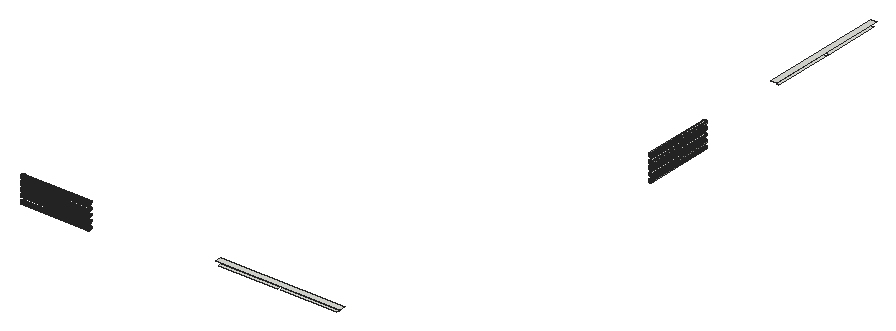
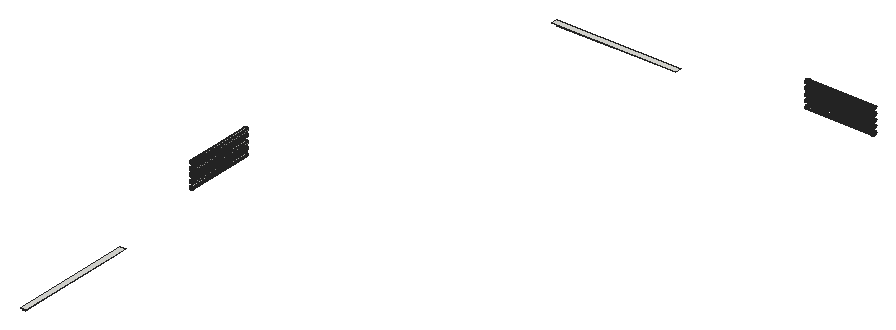
# SketchUp Ruby script. Lengths in inches.
U = 1.inch
M = Sketchup.active_model
def pt(a) = Geom::Point3d.new(a.map { |v| v * U })
def face(e, loops, mat)
  f = e.add_face(loops[0].map { |a| pt(a) })
  loops[1..].each { |l| e.add_face(l.map { |a| pt(a) }).erase! }
  f.material = f.back_material = mat if mat
  f
end
# faces: each face lists its corners as indices into pts; further lists are holes
def faces(e, pts, list, mat = nil) = list.each { |f| face(e, (f[0].is_a?(Array) ? f : [f]).map { |l| l.map { |i| pts[i] } }, mat) }
# xy, xz, yz: faces in a plane at the given z, y or x. An outline is a flat list of corners, or four numbers for a rectangle; further outlines are holes
def ring(l) = l.size == 4 ? [[l[0], l[1]], [l[2], l[1]], [l[2], l[3]], [l[0], l[3]]] : l.each_slice(2).to_a
def flat(e, list, mat, &to3) = list.each { |f| face(e, (f[0].is_a?(Array) ? f : [f]).map { |l| ring(l).map { |u, v| to3.(u, v) } }, mat) }
def xy(e, z, list, mat = nil) = flat(e, list, mat) { |x, y| [x, y, z] }
def xz(e, y, list, mat = nil) = flat(e, list, mat) { |x, z| [x, y, z] }
def yz(e, x, list, mat = nil) = flat(e, list, mat) { |y, z| [x, y, z] }
def lines(e, pts, list) = list.each { |a, b| e.add_line(pt(pts[a]), pt(pts[b])) }
# prism: a flat outline (further loops are holes) pulled along v
def prism(e, loops, v, mat = nil)
  f = face(e, loops, mat); d = Geom::Vector3d.new(v.map { |x| x * U })
  f.pushpull(f.normal.samedirection?(d) ? d.length : -d.length)
end
def box(e, o, s, mat = nil) = prism(e, [[o, [o[0] + s[0], o[1], o[2]], [o[0] + s[0], o[1] + s[1], o[2]], [o[0], o[1] + s[1], o[2]]]], [0, 0, s[2]], mat)
def at(x, y, z, deg = 0) = Geom::Transformation.translation(pt([x, y, z])) * Geom::Transformation.rotation(ORIGIN, Z_AXIS, deg.degrees)
def axes(o, x, y, z) = Geom::Transformation.new([*x, 0, *y, 0, *z, 0, *pt(o).to_a, 1])
def part(name) = M.definitions.add(name)
# library, detail: a bought-in or finely detailed component or shape, given as its bounding box
def library(name, o, s) = part(name).tap { |d| box(d.entities, o, s) }
def detail(e, o, s) = box(e.add_group.entities, o, s)
def put(e, d, t, mat = nil) = e.add_instance(d, t).tap { |i| i.material = mat if mat }
def group(e, t, mat = nil) = e.add_group.tap { |g| g.transformation = t; g.material = mat if mat }.entities
root = M.entities
xy(root,1727.61,[[1161.2,84.8125,1285.04,90.8125],[1291.04,84.8125,1408.89,90.8125],[1494,1126.01,1500,1249.86],[1494,1255.86,1500,1373.7]])
xy(root,1733.61,[[1155.2,84.8125,1414.89,96.8125],[1488,1120.01,1500,1379.7]])
p = [[922.01,48.34,1725.02],[922.01,47.38,1725.14],[778.64,47.38,1725.14],[778.64,48.34,1725.02],[922.01,49.29,1725.14],[778.64,49.29,1725.14],
  [1535.52,886.83,1725.14],[1536.47,886.83,1725.02],[1536.47,743.45,1725.02],[1535.52,743.45,1725.14],[1537.43,886.83,1725.14],[1537.43,743.45,1725.14],
  [922.01,46.5,1725.51],[778.64,46.5,1725.51],[922.01,50.18,1725.51],[778.64,50.18,1725.51],[1534.63,886.83,1725.51],[1534.63,743.45,1725.51],
  [1538.32,886.83,1725.51],[1538.32,743.45,1725.51],[922.01,45.73,1726.1],[778.64,45.73,1726.1],[922.01,50.95,1726.1],[778.64,50.95,1726.1],
  [1533.87,886.83,1726.1],[1533.87,743.45,1726.1],[1539.08,886.83,1726.1],[1539.08,743.45,1726.1],[922.01,45.15,1726.86],[778.64,45.15,1726.86],
  [922.01,51.53,1726.86],[778.64,51.53,1726.86],[1533.28,886.83,1726.86],[1533.28,743.45,1726.86],[1539.67,886.83,1726.86],[1539.67,743.45,1726.86],
  [922.01,44.78,1727.75],[778.64,44.78,1727.75],[922.01,51.9,1727.75],[778.64,51.9,1727.75],[1532.91,886.83,1727.75],[1532.91,743.45,1727.75],
  [1540.03,886.83,1727.75],[1540.03,743.45,1727.75],[922.01,44.65,1728.7],[778.64,44.65,1728.7],[922.01,52.03,1728.7],[778.64,52.03,1728.7],
  [1532.79,886.83,1728.7],[1532.79,743.45,1728.7],[1540.16,886.83,1728.7],[1540.16,743.45,1728.7],[922.01,44.78,1729.66],[778.64,44.78,1729.66],
  [922.01,51.9,1729.66],[778.64,51.9,1729.66],[1532.91,886.83,1729.66],[1532.91,743.45,1729.66],[1540.03,886.83,1729.66],[1540.03,743.45,1729.66],
  [922.01,45.15,1730.55],[778.64,45.15,1730.55],[922.01,51.53,1730.55],[778.64,51.53,1730.55],[1533.28,886.83,1730.55],[1533.28,743.45,1730.55],
  [1539.67,886.83,1730.55],[1539.67,743.45,1730.55],[922.01,45.73,1731.3125],[778.64,45.73,1731.3125],[922.01,50.95,1731.3125],[778.64,50.95,1731.3125],
  [1533.87,886.83,1731.3125],[1533.87,743.45,1731.3125],[1539.08,886.83,1731.3125],[1539.08,743.45,1731.3125],[922.01,46.5,1731.9],[778.64,46.5,1731.9],
  [922.01,50.18,1731.9],[778.64,50.18,1731.9],[1534.63,886.83,1731.9],[1534.63,743.45,1731.9],[1538.32,886.83,1731.9],[1538.32,743.45,1731.9],
  [922.01,47.38,1732.27],[778.64,47.38,1732.27],[922.01,49.29,1732.27],[778.64,49.29,1732.27],[1535.52,886.83,1732.27],[1535.52,743.45,1732.27],
  [1537.43,886.83,1732.27],[1537.43,743.45,1732.27],[922.01,48.34,1732.39],[778.64,48.34,1732.39],[1536.47,886.83,1732.39],[1536.47,743.45,1732.39],
  [922.01,48.34,1737.02],[922.01,47.38,1737.14],[778.64,47.38,1737.14],[778.64,48.34,1737.02],[922.01,49.29,1737.14],[778.64,49.29,1737.14],
  [1535.52,886.83,1737.14],[1536.47,886.83,1737.02],[1536.47,743.45,1737.02],[1535.52,743.45,1737.14],[1537.43,886.83,1737.14],[1537.43,743.45,1737.14],
  [922.01,46.5,1737.51],[778.64,46.5,1737.51],[922.01,50.18,1737.51],[778.64,50.18,1737.51],[1534.63,886.83,1737.51],[1534.63,743.45,1737.51],
  [1538.32,886.83,1737.51],[1538.32,743.45,1737.51],[922.01,45.73,1738.1],[778.64,45.73,1738.1],[922.01,50.95,1738.1],[778.64,50.95,1738.1],
  [1533.87,886.83,1738.1],[1533.87,743.45,1738.1],[1539.08,886.83,1738.1],[1539.08,743.45,1738.1],[922.01,45.15,1738.86],[778.64,45.15,1738.86],
  [922.01,51.53,1738.86],[778.64,51.53,1738.86],[1533.28,886.83,1738.86],[1533.28,743.45,1738.86],[1539.67,886.83,1738.86],[1539.67,743.45,1738.86],
  [922.01,44.78,1739.75],[778.64,44.78,1739.75],[922.01,51.9,1739.75],[778.64,51.9,1739.75],[1532.91,886.83,1739.75],[1532.91,743.45,1739.75],
  [1540.03,886.83,1739.75],[1540.03,743.45,1739.75],[922.01,44.65,1740.7],[778.64,44.65,1740.7],[922.01,52.03,1740.7],[778.64,52.03,1740.7],
  [1532.79,886.83,1740.7],[1532.79,743.45,1740.7],[1540.16,886.83,1740.7],[1540.16,743.45,1740.7],[922.01,44.78,1741.66],[778.64,44.78,1741.66],
  [922.01,51.9,1741.66],[778.64,51.9,1741.66],[1532.91,886.83,1741.66],[1532.91,743.45,1741.66],[1540.03,886.83,1741.66],[1540.03,743.45,1741.66],
  [922.01,45.15,1742.55],[778.64,45.15,1742.55],[922.01,51.53,1742.55],[778.64,51.53,1742.55],[1533.28,886.83,1742.55],[1533.28,743.45,1742.55],
  [1539.67,886.83,1742.55],[1539.67,743.45,1742.55],[922.01,45.73,1743.3125],[778.64,45.73,1743.3125],[922.01,50.95,1743.3125],[778.64,50.95,1743.3125],
  [1533.87,886.83,1743.3125],[1533.87,743.45,1743.3125],[1539.08,886.83,1743.3125],[1539.08,743.45,1743.3125],[922.01,46.5,1743.9],[778.64,46.5,1743.9],
  [922.01,50.18,1743.9],[778.64,50.18,1743.9],[1534.63,886.83,1743.9],[1534.63,743.45,1743.9],[1538.32,886.83,1743.9],[1538.32,743.45,1743.9],
  [922.01,47.38,1744.27],[778.64,47.38,1744.27],[922.01,49.29,1744.27],[778.64,49.29,1744.27],[1535.52,886.83,1744.27],[1535.52,743.45,1744.27],
  [1537.43,886.83,1744.27],[1537.43,743.45,1744.27],[922.01,48.34,1744.39],[778.64,48.34,1744.39],[1536.47,886.83,1744.39],[1536.47,743.45,1744.39],
  [922.01,48.34,1749.02],[922.01,47.38,1749.14],[778.64,47.38,1749.14],[778.64,48.34,1749.02],[922.01,49.29,1749.14],[778.64,49.29,1749.14],
  [1535.52,886.83,1749.14],[1536.47,886.83,1749.02],[1536.47,743.45,1749.02],[1535.52,743.45,1749.14],[1537.43,886.83,1749.14],[1537.43,743.45,1749.14],
  [922.01,46.5,1749.51],[778.64,46.5,1749.51],[922.01,50.18,1749.51],[778.64,50.18,1749.51],[1534.63,886.83,1749.51],[1534.63,743.45,1749.51],
  [1538.32,886.83,1749.51],[1538.32,743.45,1749.51],[922.01,45.73,1750.1],[778.64,45.73,1750.1],[922.01,50.95,1750.1],[778.64,50.95,1750.1],
  [1533.87,886.83,1750.1],[1533.87,743.45,1750.1],[1539.08,886.83,1750.1],[1539.08,743.45,1750.1],[922.01,45.15,1750.86],[778.64,45.15,1750.86],
  [922.01,51.53,1750.86],[778.64,51.53,1750.86],[1533.28,886.83,1750.86],[1533.28,743.45,1750.86],[1539.67,886.83,1750.86],[1539.67,743.45,1750.86],
  [922.01,44.78,1751.75],[778.64,44.78,1751.75],[922.01,51.9,1751.75],[778.64,51.9,1751.75],[1532.91,886.83,1751.75],[1532.91,743.45,1751.75],
  [1540.03,886.83,1751.75],[1540.03,743.45,1751.75],[922.01,44.65,1752.7],[778.64,44.65,1752.7],[922.01,52.03,1752.7],[778.64,52.03,1752.7],
  [1532.79,886.83,1752.7],[1532.79,743.45,1752.7],[1540.16,886.83,1752.7],[1540.16,743.45,1752.7],[922.01,44.78,1753.66],[778.64,44.78,1753.66],
  [922.01,51.9,1753.66],[778.64,51.9,1753.66],[1532.91,886.83,1753.66],[1532.91,743.45,1753.66],[1540.03,886.83,1753.66],[1540.03,743.45,1753.66],
  [922.01,45.15,1754.55],[778.64,45.15,1754.55],[922.01,51.53,1754.55],[778.64,51.53,1754.55],[1533.28,886.83,1754.55],[1533.28,743.45,1754.55],
  [1539.67,886.83,1754.55],[1539.67,743.45,1754.55],[922.01,45.73,1755.3125],[778.64,45.73,1755.3125],[922.01,50.95,1755.3125],[778.64,50.95,1755.3125],
  [1533.87,886.83,1755.3125],[1533.87,743.45,1755.3125],[1539.08,886.83,1755.3125],[1539.08,743.45,1755.3125],[922.01,46.5,1755.9],[778.64,46.5,1755.9],
  [922.01,50.18,1755.9],[778.64,50.18,1755.9],[1534.63,886.83,1755.9],[1534.63,743.45,1755.9],[1538.32,886.83,1755.9],[1538.32,743.45,1755.9],
  [922.01,47.38,1756.27],[778.64,47.38,1756.27],[922.01,49.29,1756.27],[778.64,49.29,1756.27],[1535.52,886.83,1756.27],[1535.52,743.45,1756.27],
  [1537.43,886.83,1756.27],[1537.43,743.45,1756.27],[922.01,48.34,1756.39],[778.64,48.34,1756.39],[1536.47,886.83,1756.39],[1536.47,743.45,1756.39],
  [922.01,48.34,1761.02],[922.01,47.38,1761.14],[778.64,47.38,1761.14],[778.64,48.34,1761.02],[922.01,49.29,1761.14],[778.64,49.29,1761.14],
  [1535.52,886.83,1761.14],[1536.47,886.83,1761.02],[1536.47,743.45,1761.02],[1535.52,743.45,1761.14],[1537.43,886.83,1761.14],[1537.43,743.45,1761.14],
  [922.01,46.5,1761.51],[778.64,46.5,1761.51],[922.01,50.18,1761.51],[778.64,50.18,1761.51],[1534.63,886.83,1761.51],[1534.63,743.45,1761.51],
  [1538.32,886.83,1761.51],[1538.32,743.45,1761.51],[922.01,45.73,1762.1],[778.64,45.73,1762.1],[922.01,50.95,1762.1],[778.64,50.95,1762.1],
  [1533.87,886.83,1762.1],[1533.87,743.45,1762.1],[1539.08,886.83,1762.1],[1539.08,743.45,1762.1],[922.01,45.15,1762.86],[778.64,45.15,1762.86],
  [922.01,51.53,1762.86],[778.64,51.53,1762.86],[1533.28,886.83,1762.86],[1533.28,743.45,1762.86],[1539.67,886.83,1762.86],[1539.67,743.45,1762.86],
  [922.01,44.78,1763.75],[778.64,44.78,1763.75],[922.01,51.9,1763.75],[778.64,51.9,1763.75],[1532.91,886.83,1763.75],[1532.91,743.45,1763.75],
  [1540.03,886.83,1763.75],[1540.03,743.45,1763.75],[922.01,44.65,1764.7],[778.64,44.65,1764.7],[922.01,52.03,1764.7],[778.64,52.03,1764.7],
  [1532.79,886.83,1764.7],[1532.79,743.45,1764.7],[1540.16,886.83,1764.7],[1540.16,743.45,1764.7],[922.01,44.78,1765.66],[778.64,44.78,1765.66],
  [922.01,51.9,1765.66],[778.64,51.9,1765.66],[1532.91,886.83,1765.66],[1532.91,743.45,1765.66],[1540.03,886.83,1765.66],[1540.03,743.45,1765.66],
  [922.01,45.15,1766.55],[778.64,45.15,1766.55],[922.01,51.53,1766.55],[778.64,51.53,1766.55],[1533.28,886.83,1766.55],[1533.28,743.45,1766.55],
  [1539.67,886.83,1766.55],[1539.67,743.45,1766.55],[922.01,45.73,1767.3125],[778.64,45.73,1767.3125],[922.01,50.95,1767.3125],[778.64,50.95,1767.3125],
  [1533.87,886.83,1767.3125],[1533.87,743.45,1767.3125],[1539.08,886.83,1767.3125],[1539.08,743.45,1767.3125],[922.01,46.5,1767.9],[778.64,46.5,1767.9],
  [922.01,50.18,1767.9],[778.64,50.18,1767.9],[1534.63,886.83,1767.9],[1534.63,743.45,1767.9],[1538.32,886.83,1767.9],[1538.32,743.45,1767.9],
  [922.01,47.38,1768.27],[778.64,47.38,1768.27],[922.01,49.29,1768.27],[778.64,49.29,1768.27],[1535.52,886.83,1768.27],[1535.52,743.45,1768.27],
  [1537.43,886.83,1768.27],[1537.43,743.45,1768.27],[922.01,48.34,1768.39],[778.64,48.34,1768.39],[1536.47,886.83,1768.39],[1536.47,743.45,1768.39],
  [922.01,48.34,1773.02],[922.01,47.38,1773.14],[778.64,47.38,1773.14],[778.64,48.34,1773.02],[922.01,49.29,1773.14],[778.64,49.29,1773.14],
  [1535.52,886.83,1773.14],[1536.47,886.83,1773.02],[1536.47,743.45,1773.02],[1535.52,743.45,1773.14],[1537.43,886.83,1773.14],[1537.43,743.45,1773.14],
  [922.01,46.5,1773.51],[778.64,46.5,1773.51],[922.01,50.18,1773.51],[778.64,50.18,1773.51],[1534.63,886.83,1773.51],[1534.63,743.45,1773.51],
  [1538.32,886.83,1773.51],[1538.32,743.45,1773.51],[922.01,45.73,1774.1],[778.64,45.73,1774.1],[922.01,50.95,1774.1],[778.64,50.95,1774.1],
  [1533.87,886.83,1774.1],[1533.87,743.45,1774.1],[1539.08,886.83,1774.1],[1539.08,743.45,1774.1],[922.01,45.15,1774.86],[778.64,45.15,1774.86],
  [922.01,51.53,1774.86],[778.64,51.53,1774.86],[1533.28,886.83,1774.86],[1533.28,743.45,1774.86],[1539.67,886.83,1774.86],[1539.67,743.45,1774.86],
  [922.01,44.78,1775.75],[778.64,44.78,1775.75],[922.01,51.9,1775.75],[778.64,51.9,1775.75],[1532.91,886.83,1775.75],[1532.91,743.45,1775.75],
  [1540.03,886.83,1775.75],[1540.03,743.45,1775.75],[922.01,44.65,1776.7],[778.64,44.65,1776.7],[922.01,52.03,1776.7],[778.64,52.03,1776.7],
  [1532.79,886.83,1776.7],[1532.79,743.45,1776.7],[1540.16,886.83,1776.7],[1540.16,743.45,1776.7],[922.01,44.78,1777.66],[778.64,44.78,1777.66],
  [922.01,51.9,1777.66],[778.64,51.9,1777.66],[1532.91,886.83,1777.66],[1532.91,743.45,1777.66],[1540.03,886.83,1777.66],[1540.03,743.45,1777.66],
  [922.01,45.15,1778.55],[778.64,45.15,1778.55],[922.01,51.53,1778.55],[778.64,51.53,1778.55],[1533.28,886.83,1778.55],[1533.28,743.45,1778.55],
  [1539.67,886.83,1778.55],[1539.67,743.45,1778.55],[922.01,45.73,1779.3125],[778.64,45.73,1779.3125],[922.01,50.95,1779.3125],[778.64,50.95,1779.3125],
  [1533.87,886.83,1779.3125],[1533.87,743.45,1779.3125],[1539.08,886.83,1779.3125],[1539.08,743.45,1779.3125],[922.01,46.5,1779.9],[778.64,46.5,1779.9],
  [922.01,50.18,1779.9],[778.64,50.18,1779.9],[1534.63,886.83,1779.9],[1534.63,743.45,1779.9],[1538.32,886.83,1779.9],[1538.32,743.45,1779.9],
  [922.01,47.38,1780.27],[778.64,47.38,1780.27],[922.01,49.29,1780.27],[778.64,49.29,1780.27],[1535.52,886.83,1780.27],[1535.52,743.45,1780.27],
  [1537.43,886.83,1780.27],[1537.43,743.45,1780.27],[922.01,48.34,1780.39],[778.64,48.34,1780.39],[1536.47,886.83,1780.39],[1536.47,743.45,1780.39]]
faces(root,p,[[0,1,2,3],[4,0,3,5],[6,7,8,9],[7,10,11,8],[1,12,13,2],[14,4,5,15],[16,6,9,17],[10,18,19,11],
  [12,20,21,13],[22,14,15,23],[24,16,17,25],[18,26,27,19],[20,28,29,21],[30,22,23,31],[32,24,25,33],[26,34,35,27],
  [28,36,37,29],[38,30,31,39],[40,32,33,41],[34,42,43,35],[36,44,45,37],[46,38,39,47],[48,40,41,49],[42,50,51,43],
  [44,52,53,45],[54,46,47,55],[56,48,49,57],[50,58,59,51],[52,60,61,53],[62,54,55,63],[64,56,57,65],[58,66,67,59],
  [60,68,69,61],[70,62,63,71],[72,64,65,73],[66,74,75,67],[68,76,77,69],[78,70,71,79],[80,72,73,81],[74,82,83,75],
  [76,84,85,77],[86,78,79,87],[88,80,81,89],[82,90,91,83],[84,92,93,85],[92,86,87,93],[94,88,89,95],[90,94,95,91],
  [96,97,98,99],[100,96,99,101],[102,103,104,105],[103,106,107,104],[97,108,109,98],[110,100,101,111],[112,102,105,113],[106,114,115,107],
  [108,116,117,109],[118,110,111,119],[120,112,113,121],[114,122,123,115],[116,124,125,117],[126,118,119,127],[128,120,121,129],[122,130,131,123],
  [124,132,133,125],[134,126,127,135],[136,128,129,137],[130,138,139,131],[132,140,141,133],[142,134,135,143],[144,136,137,145],[138,146,147,139],
  [140,148,149,141],[150,142,143,151],[152,144,145,153],[146,154,155,147],[148,156,157,149],[158,150,151,159],[160,152,153,161],[154,162,163,155],
  [156,164,165,157],[166,158,159,167],[168,160,161,169],[162,170,171,163],[164,172,173,165],[174,166,167,175],[176,168,169,177],[170,178,179,171],
  [172,180,181,173],[182,174,175,183],[184,176,177,185],[178,186,187,179],[180,188,189,181],[188,182,183,189],[190,184,185,191],[186,190,191,187],
  [192,193,194,195],[196,192,195,197],[198,199,200,201],[199,202,203,200],[193,204,205,194],[206,196,197,207],[208,198,201,209],[202,210,211,203],
  [204,212,213,205],[214,206,207,215],[216,208,209,217],[210,218,219,211],[212,220,221,213],[222,214,215,223],[224,216,217,225],[218,226,227,219],
  [220,228,229,221],[230,222,223,231],[232,224,225,233],[226,234,235,227],[228,236,237,229],[238,230,231,239],[240,232,233,241],[234,242,243,235],
  [236,244,245,237],[246,238,239,247],[248,240,241,249],[242,250,251,243],[244,252,253,245],[254,246,247,255],[256,248,249,257],[250,258,259,251],
  [252,260,261,253],[262,254,255,263],[264,256,257,265],[258,266,267,259],[260,268,269,261],[270,262,263,271],[272,264,265,273],[266,274,275,267],
  [268,276,277,269],[278,270,271,279],[280,272,273,281],[274,282,283,275],[276,284,285,277],[284,278,279,285],[286,280,281,287],[282,286,287,283],
  [288,289,290,291],[292,288,291,293],[294,295,296,297],[295,298,299,296],[289,300,301,290],[302,292,293,303],[304,294,297,305],[298,306,307,299],
  [300,308,309,301],[310,302,303,311],[312,304,305,313],[306,314,315,307],[308,316,317,309],[318,310,311,319],[320,312,313,321],[314,322,323,315],
  [316,324,325,317],[326,318,319,327],[328,320,321,329],[322,330,331,323],[324,332,333,325],[334,326,327,335],[336,328,329,337],[330,338,339,331],
  [332,340,341,333],[342,334,335,343],[344,336,337,345],[338,346,347,339],[340,348,349,341],[350,342,343,351],[352,344,345,353],[346,354,355,347],
  [348,356,357,349],[358,350,351,359],[360,352,353,361],[354,362,363,355],[356,364,365,357],[366,358,359,367],[368,360,361,369],[362,370,371,363],
  [364,372,373,365],[374,366,367,375],[376,368,369,377],[370,378,379,371],[372,380,381,373],[380,374,375,381],[382,376,377,383],[378,382,383,379],
  [384,385,386,387],[388,384,387,389],[390,391,392,393],[391,394,395,392],[385,396,397,386],[398,388,389,399],[400,390,393,401],[394,402,403,395],
  [396,404,405,397],[406,398,399,407],[408,400,401,409],[402,410,411,403],[404,412,413,405],[414,406,407,415],[416,408,409,417],[410,418,419,411],
  [412,420,421,413],[422,414,415,423],[424,416,417,425],[418,426,427,419],[420,428,429,421],[430,422,423,431],[432,424,425,433],[426,434,435,427],
  [428,436,437,429],[438,430,431,439],[440,432,433,441],[434,442,443,435],[436,444,445,437],[446,438,439,447],[448,440,441,449],[442,450,451,443],
  [444,452,453,445],[454,446,447,455],[456,448,449,457],[450,458,459,451],[452,460,461,453],[462,454,455,463],[464,456,457,465],[458,466,467,459],
  [460,468,469,461],[470,462,463,471],[472,464,465,473],[466,474,475,467],[468,476,477,469],[476,470,471,477],[478,472,473,479],[474,478,479,475]])
